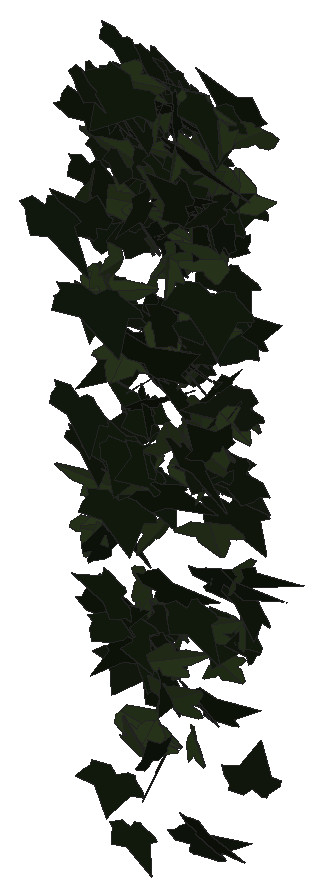
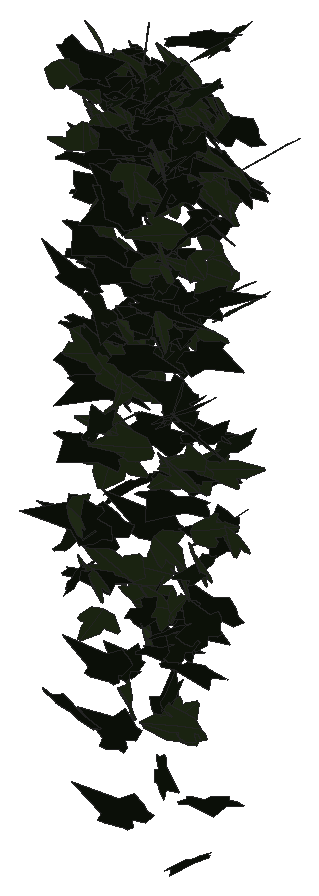
# SketchUp Ruby script. Lengths in millimetres.
U = 1.mm
M = Sketchup.active_model
def pt(a) = Geom::Point3d.new(a.map { |v| v * U })
def face(e, loops, mat)
  f = e.add_face(loops[0].map { |a| pt(a) })
  loops[1..].each { |l| e.add_face(l.map { |a| pt(a) }).erase! }
  f.material = f.back_material = mat if mat
  f
end
# faces: each face lists its corners as indices into pts; further lists are holes
def faces(e, pts, list, mat = nil) = list.each { |f| face(e, (f[0].is_a?(Array) ? f : [f]).map { |l| l.map { |i| pts[i] } }, mat) }
# xy, xz, yz: faces in a plane at the given z, y or x. An outline is a flat list of corners, or four numbers for a rectangle; further outlines are holes
def ring(l) = l.size == 4 ? [[l[0], l[1]], [l[2], l[1]], [l[2], l[3]], [l[0], l[3]]] : l.each_slice(2).to_a
def flat(e, list, mat, &to3) = list.each { |f| face(e, (f[0].is_a?(Array) ? f : [f]).map { |l| ring(l).map { |u, v| to3.(u, v) } }, mat) }
def xy(e, z, list, mat = nil) = flat(e, list, mat) { |x, y| [x, y, z] }
def xz(e, y, list, mat = nil) = flat(e, list, mat) { |x, z| [x, y, z] }
def yz(e, x, list, mat = nil) = flat(e, list, mat) { |y, z| [x, y, z] }
def lines(e, pts, list) = list.each { |a, b| e.add_line(pt(pts[a]), pt(pts[b])) }
# prism: a flat outline (further loops are holes) pulled along v
def prism(e, loops, v, mat = nil)
  f = face(e, loops, mat); d = Geom::Vector3d.new(v.map { |x| x * U })
  f.pushpull(f.normal.samedirection?(d) ? d.length : -d.length)
end
def box(e, o, s, mat = nil) = prism(e, [[o, [o[0] + s[0], o[1], o[2]], [o[0] + s[0], o[1] + s[1], o[2]], [o[0], o[1] + s[1], o[2]]]], [0, 0, s[2]], mat)
def at(x, y, z, deg = 0) = Geom::Transformation.translation(pt([x, y, z])) * Geom::Transformation.rotation(ORIGIN, Z_AXIS, deg.degrees)
def axes(o, x, y, z) = Geom::Transformation.new([*x, 0, *y, 0, *z, 0, *pt(o).to_a, 1])
def part(name) = M.definitions.add(name)
# library, detail: a bought-in or finely detailed component or shape, given as its bounding box
def library(name, o, s) = part(name).tap { |d| box(d.entities, o, s) }
def detail(e, o, s) = box(e.add_group.entities, o, s)
def put(e, d, t, mat = nil) = e.add_instance(d, t).tap { |i| i.material = mat if mat }
def group(e, t, mat = nil) = e.add_group.tap { |g| g.transformation = t; g.material = mat if mat }.entities
root = M.entities
M.materials.add("efeu1").color = [18, 25, 13]
M.materials.add("efeu2").color = [43, 57, 29]
c1 = part("ivyleaf_9")
p = [[39.1,54.8,31.7],[34.5,51.8,30.2],[-5.3,25.2,17.3],[-17.9,28.3,20.9],[-21.6,21.7,17],[-20.2,4.3,5.3],
  [-22.9,-0.3,2.5],[-17.1,-4,-0.6],[-2,-2.1,-1.2],[-0.7,-15.4,-10.1],[16.6,-22.3,-16.7],[21.1,-15.1,-12.5],
  [32.7,-10.7,-11],[46.1,-1.8,-6.6],[30.8,11.2,3.8]]
faces(c1.entities,p,[[0,1,2,3,4,5,6,7,8,9,10,11,12,13,14]],"efeu1")
c2 = part("ivyleaf_10")
p = [[0,12.8,-0.8],[-1.5,51.3,-10.9],[-4.9,51,-11.6],[-13.6,26.5,-7.3],[-13.2,15.9,-4.6],[-21.1,19.3,-7.2],
  [-29.5,16.3,-8.3],[-29.2,8.3,-6.2],[-19.7,-9.8,0.5],[-7.6,-13,4],[1,-12.2,5.8],[-0.4,51.1,-11.1],
  [-1.5,51.1,-10.9],[1,-12.4,5.9],[16.9,-12.4,3.5],[35.1,9.1,-5.1],[35,12.9,-6.1],[20.5,16.4,-4.9],
  [15.8,15,-3.8],[15.3,27.6,-7.1],[12.8,31.3,-7.8]]
faces(c2.entities,p,[[0,1,2,3,4,5,6,7,8,9,10],[11,12,0,13,14,15,16,17,18,19,20]],"efeu2")
put(root,c1,axes([3148,691.4,1357.3],[-1.09848,-0.61121,-0.72388],[0.90904,0.5443,-0.84042],[1.55717,-0.74891,-0.02003]))
put(root,c1,axes([3099.4,712.5,1161.4],[-0.04032,-1.07026,0.20723],[-0.0125,-0.20714,-1.07047],[2.07471,-0.02205,-0.00242]))
put(root,c1,axes([3032,722.5,1449.5],[0.63761,-1.12764,-0.34099],[-0.10545,0.33903,-1.17561],[2.23961,0.337,0.04172]))
put(root,c2,axes([3239.9,749.2,1415.5],[0.02125,0.68623,-0.62586],[-0.04877,-0.62544,-0.68623],[-1.76696,0.02552,0.01141]))
put(root,c1,axes([3194.2,748.7,1503.5],[-1.17443,0.48349,-0.48625],[0.73727,-0.29397,-0.78391],[-1.07685,-0.72857,-0.00639]))
put(root,c1,axes([3272.7,736.2,1533.3],[-0.8878,0.19774,-0.78509],[-1.49185,0.11635,0.49506],[0.38545,0.90577,0.10781]))
put(root,c1,axes([3175.7,773.9,1222.5],[-0.44551,-0.12491,0.99895],[1.62914,-0.56451,0.13],[1.00847,0.85676,0.2313]))
put(root,c1,axes([3253.8,772.5,840.3],[0.29351,-0.90626,-0.43034],[-0.16178,0.42203,-0.91922],[1.90251,0.1757,-0.01177]))
put(root,c1,axes([3088.2,761.2,1424.8],[-0.46198,0.35449,0.80046],[-0.83868,0.66827,-0.42959],[-1.43967,-0.50306,-0.00661]))
put(root,c1,axes([3063.1,778.3,1657.5],[0.90349,-0.93415,-0.35024],[-0.25619,0.32435,-1.04754],[1.88137,0.49278,0.02555]))
put(root,c1,axes([3108.5,793.1,802.7],[0.10206,-0.93985,-0.20129],[0.12799,-0.19744,0.93979],[-1.8248,-0.06641,0.05466]))
put(root,c1,axes([3124.6,800,1646.3],[-1.33312,-0.81117,0.30777],[-0.35091,-0.24734,-1.07154],[1.61349,-0.72401,0.02124]))
put(root,c2,axes([3277,792.5,1420.5],[0.89623,0.07208,-0.78678],[-1.49317,-0.06543,-0.47557],[-0.17745,0.9146,0.02799]))
put(root,c2,axes([3207.7,792.5,668.4],[-1.45962,-0.06032,0.58543],[1.11508,0.01263,0.76884],[-0.10585,0.96475,0.02654]))
put(root,c1,axes([3188.6,813.3,681.3],[0.36799,-0.32379,-0.95206],[1.23033,-0.70261,0.37024],[-1.46603,-0.67093,0.07174]))
put(root,c2,axes([3200.4,811.8,1398.7],[0.20071,-0.42785,0.89084],[0.32043,-0.87502,-0.44019],[1.85335,0.19762,-0.02037]))
put(root,c1,axes([3271.3,806.9,1097.5],[0.4774,0.30872,0.88717],[-1.31395,-0.56208,0.3908],[1.21229,-0.73079,0.0742]))
put(root,c1,axes([3218.8,804.7,1078.1],[0.96684,-0.9688,0.10046],[0.09693,-0.08672,-1.0939],[1.85117,0.51053,0.00481]))
put(root,c2,axes([3156.7,808.8,1496.4],[-0.24848,-0.06951,1.03991],[1.78685,-0.46289,0.08693],[0.86124,0.94032,0.11967]))
put(root,c1,axes([3203.5,791.6,1287.1],[-0.51143,0.05826,-0.9062],[-1.71549,0.09747,0.27355],[0.20954,0.94016,0.0278]))
put(root,c1,axes([3264.3,811.5,1344.9],[-1.0371,-0.88274,-0.40095],[0.4247,0.3334,-1.0373],[1.79567,-0.58869,0.01376]))
put(root,c2,axes([3081.2,820.5,1337.4],[-0.03831,0.03747,0.8963],[0.47235,-0.8613,0.04159],[1.6407,0.24884,0.00896]))
put(root,c1,axes([3173,815.5,1390.4],[0.03374,-0.02831,0.98933],[0.79772,-0.89616,-0.03315],[1.7064,0.4195,-0.00406]))
put(root,c2,axes([3051.7,816.1,1311],[0.85802,-0.35978,0.67627],[1.14747,-0.31739,-0.57078],[0.8993,0.74824,0.08306]))
put(root,c1,axes([3036.7,823.7,1255.8],[-0.31691,-0.83164,0.26203],[-0.10244,-0.25646,-0.84814],[1.65632,-0.17498,-0.00232]))
put(root,c1,axes([3140.3,830.4,1011.4],[-0.57944,-0.40887,0.87701],[-0.74051,-0.79006,-0.50341],[1.68616,-0.48748,0.0803]))
put(root,c2,axes([3188.2,795,722.8],[-0.15978,-0.32421,0.94485],[0.70743,0.86995,0.33153],[-1.76463,0.37812,0.04736]))
put(root,c1,axes([3284.6,810.4,1499.4],[-1.11102,0.68743,-0.20394],[0.25146,-0.15535,-0.90186],[-1.34131,-0.59853,-0.00015]))
put(root,c1,axes([3020.5,835.2,1001.4],[-0.08767,-0.80776,0.5954],[0.1958,-0.59669,-0.80155],[1.89976,0.02422,0.11009]))
put(root,c1,axes([3229.5,826.6,441],[0.54603,-0.41934,0.71364],[0.83487,-0.56347,-0.50746],[1.3359,0.52354,0.02545]))
put(root,c1,axes([3084.2,824.3,936.9],[-0.74249,-0.83718,-0.37572],[0.27869,0.34623,-0.92354],[1.72405,-0.41652,-0.01252]))
put(root,c2,axes([3169.2,811.5,1261.3],[0.56052,0.80983,0.27461],[0.20124,0.25372,-0.86164],[-1.61498,0.31269,-0.01206]))
put(root,c1,axes([3102.9,826.8,1021.5],[-1.48522,-0.20119,-0.38935],[0.72941,0.07237,-0.80557],[0.40456,-0.86911,0.02305]))
put(root,c2,axes([3055.3,826.7,957],[-0.50076,-0.05485,-0.84838],[-1.5783,-0.17897,0.26877],[-0.35623,0.87002,0.0018]))
put(root,c2,axes([3187.8,832.2,1550.4],[-0.00871,0.65938,-0.65939],[-0.13524,-0.65773,-0.65722],[-1.76959,0.04702,0.05347]))
put(root,c2,axes([3032.1,816.5,1449.1],[0.03873,-0.99592,-0.42809],[0.11975,0.42852,-0.99395],[2.05964,-0.00619,0.06584]))
put(root,c1,axes([3200.2,817.5,1443.3],[-0.67275,0.83089,-0.13837],[0.10765,-0.1263,-0.90296],[-1.59952,-0.35797,-0.00257]))
put(root,c2,axes([3274.8,816.8,1073.7],[0.3277,-0.05341,0.90413],[-1.69,0.17123,0.17922],[-0.33935,-0.90431,-0.01946]))
put(root,c1,axes([3197.4,810.1,1632],[0.50681,-0.22295,-0.94817],[-1.4527,0.56287,-0.34672],[1.15159,0.80816,-0.02009]))
put(root,c1,axes([3156.5,826.7,814.8],[0.26163,-0.08827,0.88895],[1.40149,-0.49797,-0.16332],[0.96249,0.7491,-0.00382]))
put(root,c1,axes([3191.8,810.2,1482],[1.32216,0.55374,0.20711],[0.31203,0.12659,-0.88838],[-1.08105,0.71378,-0.00312]))
put(root,c1,axes([3186.8,827.5,1552.9],[1.58032,-0.52072,0.48441],[0.79507,-0.24554,-0.98004],[1.09544,0.92943,0.01248]))
put(root,c1,axes([3099.7,838.4,1182],[1.22544,-0.25384,-0.75639],[1.39495,-0.19579,0.68964],[-0.59987,-0.97385,0.05851]))
put(root,c1,axes([3285.3,812.6,1441.6],[0.26022,-0.08442,0.91084],[-0.26081,0.90868,0.10479],[-1.7213,-0.15045,0.12182]))
put(root,c1,axes([3091.9,839.6,695.2],[-0.25426,0.27227,-0.80449],[0.3543,-0.78519,-0.29666],[-1.57711,-0.22029,0.06306]))
put(root,c2,axes([3110.2,845,1392.7],[-0.51743,-0.16957,1.02457],[1.56141,-0.68442,0.10443],[1.21182,0.80946,0.30292]))
put(root,c1,axes([3155.1,817.3,982.5],[0.0257,0.1341,-0.89414],[0.52498,0.85099,0.1318],[1.63872,-0.27473,-0.0282]))
put(root,c1,axes([3114,822.9,1227.1],[1.53416,0.39429,-0.53653],[-0.93512,-0.21633,-0.89717],[-0.85521,0.94385,0.01851]))
put(root,c1,axes([3123.1,828,1387.6],[-1.26853,0.56479,0.32275],[-0.48523,0.19832,-0.87354],[-1.13899,-0.71351,0.01268]))
put(root,c2,axes([3166.5,841.7,1051.8],[-0.82199,-0.82846,-0.30957],[-0.28298,-0.27159,0.93426],[-1.65924,0.45674,-0.00598]))
put(root,c1,axes([3071.7,847.3,1155.3],[-0.08561,0.08958,-0.88875],[0.18329,-0.88421,-0.094],[-1.69014,-0.10043,0.03482]))
put(root,c2,axes([3084.1,836.3,1176.7],[1.51571,0.3624,-0.22264],[-0.38648,-0.09129,-0.87498],[-0.71127,0.82188,0.00098]))
put(root,c1,axes([3131.6,843.6,520.5],[0.53627,0.37491,0.77182],[-0.8286,-0.63757,0.46864],[1.40723,-0.51828,-0.01819]))
put(root,c1,axes([3018,839.5,1463.6],[-0.89889,-0.013,-0.75126],[1.42369,0.07519,-0.47159],[0.13428,-0.8842,-0.02906]))
put(root,c2,axes([3048,823.7,1276.7],[0.53546,0.15131,-1.02625],[1.82124,0.37262,0.31728],[0.76213,-0.99675,-0.03717]))
put(root,c1,axes([3206.1,833.6,1228.6],[-0.68489,0.53399,0.64734],[0.72924,-0.52209,0.64367],[1.42089,0.52534,-0.01832]))
put(root,c2,axes([3207,840.9,1086.5],[-0.00156,-0.2175,0.94094],[1.82422,-0.11521,-0.0258],[0.2247,0.93386,0.21596]))
put(root,c1,axes([3303,837.1,1056],[-0.1535,-0.02592,-1.05543],[-1.77978,-0.48951,0.08348],[-0.93253,0.93851,0.0144]))
put(root,c2,axes([3020.6,840.6,867.1],[1.41101,-0.46828,0.11897],[0.19326,-0.06201,-0.87689],[0.899,0.74831,0.00178]))
put(root,c2,axes([3279.4,823,1593.2],[0.7223,-0.12595,0.85868],[-1.0972,0.66396,0.35219],[-1.23465,-0.66372,0.18937]))
put(root,c1,axes([3011.3,840.2,1537.7],[-0.58251,0.12731,0.95543],[1.49699,-0.54641,0.32478],[1.06029,0.8414,0.06636]))
put(root,c2,axes([3208.4,842,1264.8],[0.75904,-0.19884,-0.90022],[1.64876,-0.25468,0.44005],[-0.60018,-0.95111,0.07037]))
put(root,c1,axes([3040.4,820.9,845],[0.19601,0.1337,1.01729],[1.32206,0.74337,-0.16803],[-1.43716,0.70206,-0.01582]))
put(root,c2,axes([3049.6,836.3,1424.3],[-0.50917,-0.08974,0.92934],[1.65127,0.33321,0.28194],[-0.6564,0.90786,-0.01162]))
put(root,c1,axes([3070.5,842.8,727],[-0.2822,-0.74749,-0.57441],[0.41705,0.53822,-0.75695],[1.745,-0.24951,0.08802]))
put(root,c2,axes([3159.4,853.4,655.9],[0.36921,-0.80251,0.49862],[0.22163,-0.48483,-0.82562],[1.78443,0.22626,-0.00062]))
put(root,c1,axes([3062.8,848.1,1603.8],[-1.12509,0.16505,-0.63443],[1.17807,-0.14072,-0.61339],[-0.41077,-0.85567,-0.0215]))
put(root,c2,axes([3063.5,844.2,1437],[1.79211,-0.26869,-0.48567],[-0.8916,0.12818,-0.97921],[0.56651,1.05172,-0.00474]))
put(root,c1,axes([3053.3,863.3,1255.6],[-0.1669,-0.5801,-0.82183],[-0.01178,-0.82462,0.58273],[-1.91447,0.05565,0.06806]))
put(root,c1,axes([3054.3,830.3,1379.4],[0.21308,-0.12772,-0.87621],[-0.14631,0.87845,-0.13787],[1.67887,0.09277,0.09919]))
put(root,c1,axes([3073,842.9,1004.7],[-1.1688,-0.59294,0.28239],[0.40465,0.1863,0.85355],[-1.18261,0.64976,0.01297]))
put(root,c1,axes([3274.7,858.6,1264.6],[-0.54401,-0.45618,-0.90021],[-0.78855,-0.80009,0.53701],[-1.75137,0.50194,0.03784]))
put(root,c1,axes([3252.4,849.3,1053.9],[-1.47449,0.23162,-0.36199],[0.6657,-0.0937,-0.80857],[-0.47519,-0.84999,-0.00951]))
put(root,c1,axes([3033.6,848.7,722.3],[-0.25491,0.09954,0.9014],[1.23283,-0.62719,0.16551],[1.20794,0.66112,0.0213]))
put(root,c1,axes([3085,836.8,1401],[-1.13867,0.58624,0.31908],[0.4534,-0.21271,0.83752],[1.18662,0.64383,-0.01383]))
put(root,c1,axes([3129.5,866.2,1251.4],[0.93687,-0.85042,-0.4558],[0.68274,-0.31371,0.97273],[-1.70471,-0.59301,0.13908]))
put(root,c2,axes([3204.7,852.2,1536.4],[-0.30219,-0.08567,1.02244],[-1.82264,-0.35892,-0.17879],[0.70077,-0.97045,-0.02413]))
put(root,c1,axes([3105.6,842.2,1129.4],[0.38507,0.86361,0.15474],[-0.09303,-0.14746,0.88689],[1.66721,-0.20769,0.01375]))
put(root,c1,axes([3084.6,864.8,1563],[-0.18898,-0.82758,0.41164],[0.33627,-0.42337,-0.80854],[1.7267,-0.00812,0.20251]))
put(root,c2,axes([3077.5,859.6,1619],[0.59979,-0.26489,-0.90917],[1.33262,-0.57992,0.41167],[-1.21338,-0.76785,0.00272]))
put(root,c2,axes([3125.5,862.4,1584.3],[0.80852,-0.62316,0.5523],[0.64367,-0.43745,-0.75371],[1.44816,0.54235,0.02665]))
put(root,c1,axes([3132.8,860.9,1229.7],[0.75214,-0.64198,0.51276],[0.67123,-0.38135,-0.74928],[1.41231,0.52314,0.08304]))
put(root,c2,axes([3106.8,846.8,525],[-1.14631,0.5595,-0.36444],[-0.5126,0.24553,0.82208],[1.16285,0.65978,0.00312]))
put(root,c1,axes([3236.9,847.4,1044.9],[0.01688,-0.57967,-0.91706],[0.51885,0.88886,-0.5592],[1.99854,-0.22587,0.15292]))
put(root,c2,axes([3044.1,872.3,873.7],[-0.18463,0.03472,0.93901],[-0.23888,-0.93602,0.02164],[1.77232,-0.12254,0.10074]))
put(root,c2,axes([3258.3,846.5,1295.2],[-0.42523,-0.76212,-0.59809],[0.36332,0.56712,-0.79397],[1.80763,-0.29327,0.01889]))
put(root,c1,axes([3237.7,873.8,1451.7],[-0.42162,-0.82284,0.36012],[-0.17519,-0.34816,-0.85214],[1.70043,-0.23989,0.0015]))
put(root,c1,axes([3182.5,870.2,1513],[-0.19489,-0.94627,0.07143],[-0.0095,-0.0713,-0.95179],[1.80604,-0.10248,0.0027]))
put(root,c2,axes([3169.8,871.5,1469.9],[0.58916,-0.37685,0.75157],[0.9217,-0.57476,-0.48767],[1.30801,0.57475,0.00511]))
put(root,c1,axes([3105.7,855.8,1592.1],[1.40563,-0.2124,0.4587],[0.84346,-0.11856,-0.76846],[0.46274,0.86129,0.00734]))
put(root,c1,axes([3143.7,870.8,1184.6],[0.62085,-0.63434,0.56384],[0.44542,-0.5134,-0.713],[1.55263,0.40094,-0.02092]))
put(root,c2,axes([3106.5,854.4,796.9],[0.82241,-0.80605,-0.48884],[-0.33384,0.45961,-0.91291],[1.76281,0.46309,0.05517]))
put(root,c1,axes([3220.3,873.1,1614],[-0.49748,-1.01728,-0.03229],[0.01648,0.03112,-1.05033],[1.93699,-0.26153,0.00064]))
put(root,c2,axes([3135.6,859.5,1590.4],[1.02429,-0.65135,-0.26115],[-0.27666,0.21849,-0.84454],[1.30662,0.55688,0.0259]))
put(root,c2,axes([3227.1,857.6,928.6],[-1.59016,-0.50603,-0.18202],[0.29431,0.09602,-0.97681],[0.98026,-0.84971,-0.00199]))
put(root,c2,axes([3264.7,849,1126.9],[0.1426,0.79738,0.51971],[0.06277,0.51883,-0.80078],[-1.81036,0.0808,0.01317]))
put(root,c1,axes([3060.7,869,1612],[-0.15584,-0.91483,-0.23042],[0.05705,0.22865,-0.91844],[1.79458,-0.08671,0.00919]))
put(root,c1,axes([3093.9,874.4,953.4],[-1.22073,-0.55624,0.03278],[-0.04578,-0.02229,-0.84901],[1.05948,-0.64186,0.00108]))
put(root,c1,axes([3131.9,878.5,1129.2],[0.33649,-0.87178,0.44567],[0.26842,-0.42548,-0.88823],[1.84397,0.22102,0.04797]))
put(root,c2,axes([3081.2,852.3,957.9],[-0.96001,-0.44969,-0.84006],[1.21341,0.5471,-0.67569],[1.3477,-0.81291,0.00996]))
put(root,c2,axes([3063.4,858.6,1495.2],[0.10711,-0.01039,0.99452],[-1.87733,0.12679,0.05715],[-0.24205,-0.98801,-0.00313]))
put(root,c2,axes([3212.5,881.8,1000.9],[0.30462,-0.49896,0.81623],[0.42544,-0.78516,-0.5238],[1.77031,0.27455,-0.01457]))
put(root,c1,axes([3060.9,872.1,1612.1],[-1.20176,0.09243,-0.60215],[1.12769,-0.10835,-0.63798],[-0.26942,-0.86577,0.01556]))
put(root,c1,axes([3282.1,872.2,1140.6],[-1.4112,-0.04215,0.44705],[-0.85123,-0.00721,-0.74252],[0.07579,-0.8658,-0.01558]))
put(root,c1,axes([3159.2,868,1257.6],[1.20713,-0.34664,0.57854],[0.95845,-0.28486,-0.72278],[0.85381,0.80985,-0.0066]))
put(root,c2,axes([3164.7,870,1450.2],[-1.18883,0.0604,-0.75787],[-1.44662,-0.02901,0.62418],[0.03039,0.98168,0.06508]))
put(root,c1,axes([3108.6,868.4,1198.9],[1.44661,-0.39648,0.29598],[0.49928,-0.13706,-0.85728],[0.79839,0.80409,-0.00018]))
put(root,c1,axes([3246.1,848.6,1166.5],[0.16897,0.71867,0.61151],[0.1303,0.60768,-0.72412],[-1.79118,0.112,0.00501]))
put(root,c2,axes([3248.7,870.5,1508],[1.382,-0.72293,-0.12259],[-0.13676,0.10154,-1.02444],[1.38881,0.72939,0.02111]))
put(root,c1,axes([3225.7,879,1375.3],[0.96986,0.22223,0.84296],[-1.46209,-0.34706,0.55591],[0.78425,-0.92185,-0.00607]))
put(root,c1,axes([3034.9,887.5,1557.9],[0.03908,-0.73537,0.56993],[-0.01775,-0.57021,-0.73539],[1.7706,0.01051,-0.01995]))
put(root,c1,axes([3106.2,866.7,1477.5],[-0.26339,0.22561,0.8065],[-1.33853,0.41247,-0.23607],[-0.86529,-0.70673,0.11968]))
put(root,c2,axes([3174.2,873.7,1606],[-0.0944,0.00486,-0.90035],[1.63504,-0.2696,-0.04878],[-0.51282,-0.86047,0.0102]))
put(root,c1,axes([3057.4,875.4,1568.8],[-1.36606,0.27318,-0.35069],[0.64422,-0.09588,-0.76749],[-0.54843,-0.79309,-0.02801]))
put(root,c1,axes([3083,888.1,1079.4],[0.34647,-0.15233,-0.90399],[1.34867,-0.56132,0.23729],[-1.10688,-0.73162,0.00616]))
put(root,c2,axes([3197.2,869.8,749.6],[-1.19274,-0.30094,0.6971],[1.21052,0.28557,0.6951],[-0.78921,0.89283,0.01264]))
put(root,c1,axes([3083.7,878.4,1561.7],[-0.25442,-0.94281,-0.35649],[0.18901,0.34554,-0.9511],[1.90901,-0.15987,0.04666]))
put(root,c2,axes([3103.6,878.1,1289.8],[0.5209,-0.76664,-0.23931],[0.1543,-0.22515,0.81403],[-1.52069,-0.28545,0.00062]))
put(root,c1,axes([3257.3,876.9,1139.9],[-0.99973,0.5187,-0.44741],[0.56591,-0.33527,-0.73779],[-1.17446,-0.60308,0.02535]))
put(root,c2,axes([3074.4,856.2,960.2],[-0.0229,-0.38747,0.96378],[0.05174,0.9634,0.38766],[-1.97628,0.02971,-0.00102]))
put(root,c1,axes([3069.8,866.9,1537.2],[1.42122,-0.11122,-0.47303],[-0.88584,0.08547,-0.75487],[0.26571,0.87983,0.01353]))
put(root,c2,axes([3167.4,887.7,547.1],[0.22037,-0.11647,0.92285],[1.32418,-0.60639,-0.16383],[1.17497,0.70524,0.01155]))
put(root,c2,axes([3170.4,868.5,1147.1],[0.40976,-0.80851,0.35731],[-0.00132,0.3676,0.83222],[-1.68232,-0.19722,0.08638]))
put(root,c2,axes([3227.1,880.7,1500.8],[-0.39561,-0.89241,0.2302],[0.00526,-0.23659,-0.91467],[1.75402,-0.20057,0.05466]))
put(root,c2,axes([3033.3,859.9,1580.3],[-0.38709,-0.20216,-0.98043],[1.30495,0.7008,-0.28674],[1.38813,-0.71518,-0.00384]))
put(root,c1,axes([3100.5,880,690.6],[-0.87332,-0.06523,-0.85105],[1.58611,0.17448,-0.46272],[0.3509,-0.951,-0.02653]))
put(root,c1,axes([3134.3,858.7,1589.5],[0.95335,0.40394,0.56191],[0.71034,0.42644,-0.63928],[-1.10911,0.62033,0.07357]))
put(root,c1,axes([3141.1,871.4,1508.1],[0.41935,-0.57747,-0.68822],[0.46665,0.72037,-0.52594],[1.64492,-0.05715,0.32466]))
put(root,c2,axes([3119,885.6,1495.8],[0.16882,-0.87143,0.33371],[0.08431,-0.3309,-0.87588],[1.77395,0.09866,0.00987]))
put(root,c1,axes([3066.4,885.9,645.9],[-1.37329,-0.40686,-0.14062],[0.2364,0.066,-0.82836],[0.78443,-0.73217,0.00347]))
put(root,c2,axes([3138.9,889.6,691.5],[0.54017,-0.62548,0.57367],[0.50051,-0.51032,-0.68651],[1.53579,0.38631,0.02196]))
put(root,c1,axes([3062.6,868.5,1491.2],[0.48476,-0.54872,-0.85661],[-0.30208,0.8508,-0.59219],[1.91238,0.27348,0.12359]))
put(root,c1,axes([3195.7,874.4,1441.3],[-0.3702,-0.02702,0.88712],[1.66102,-0.17085,0.18616],[0.30693,0.89198,0.06253]))
put(root,c1,axes([3147.7,889.9,1466.4],[-1.72751,-0.27954,0.29998],[-0.54718,-0.08564,-0.94975],[0.55641,-0.95213,-0.00265]))
put(root,c1,axes([3080.1,866,1075.6],[0.44392,0.84885,-0.28298],[0.13865,0.27345,0.88031],[1.69729,-0.24435,0.0021]))
put(root,c1,axes([3026,888.5,435.1],[-0.90851,-0.66946,-0.11372],[0.13134,0.09046,-0.82221],[1.28567,-0.48231,0.00364]))
put(root,c1,axes([3089.6,880.1,1049.2],[-1.49317,0.3526,0.08163],[-0.14448,0.03021,-0.86014],[-0.67349,-0.78821,0.00355]))
put(root,c1,axes([3142.7,886,1227.3],[-1.38722,0.02884,0.51759],[-0.98611,-0.01249,-0.72896],[-0.03097,-0.89388,0.02688]))
put(root,c1,axes([3099.2,885.2,1049],[-0.75033,-0.86849,0.10666],[0.08337,0.09724,0.95379],[-1.66324,0.39667,-0.00031]))
put(root,c2,axes([3197.5,871,1550.3],[0.58517,-0.52133,-0.65044],[-0.46316,0.60694,-0.6015],[1.51736,0.38631,0.06725]))
put(root,c2,axes([3086,878.4,516],[1.53144,0.10699,-0.20891],[0.39234,0.03455,0.81172],[0.21357,-0.83063,0.00685]))
put(root,c2,axes([3180.6,871.9,1086.7],[-0.36234,-0.733,-0.64026],[0.41278,0.60404,-0.75602],[1.80572,-0.28517,0.04434]))
put(root,c1,axes([3163.5,896.2,610.7],[0.27611,-0.47662,0.66592],[0.44391,-0.62423,-0.49759],[1.49399,0.27356,0.02478]))
put(root,c1,axes([3045.8,881.9,1386.2],[0.53809,-0.72917,-0.45243],[-0.33134,0.4177,-0.78201],[1.59922,0.33189,-0.00979]))
put(root,c1,axes([3013.1,879.8,1484.9],[0.75256,-0.67732,-0.47211],[-0.06145,0.51038,-0.75926],[1.57012,0.34461,0.19657]))
put(root,c2,axes([3163.4,895,1393.2],[-0.35089,0.10656,0.9668],[1.53869,-0.5303,0.21262],[1.02919,0.82915,0.01174]))
put(root,c2,axes([3190,884.7,993.3],[0.07829,-0.10916,0.8964],[1.71248,0.08079,-0.03146],[-0.14524,0.8937,0.11234]))
put(root,c2,axes([3184.8,886.9,1085.7],[-0.81757,-0.05843,0.8945],[1.70315,0.02971,0.43171],[-0.09917,0.99186,0.03976]))
put(root,c1,axes([3098.4,895.6,667.7],[-0.92556,-0.72464,-0.09334],[0.09629,0.07845,-0.8727],[1.38719,-0.48894,-0.0017]))
put(root,c1,axes([3129.8,901.5,729.1],[-0.10043,-0.10494,-0.85907],[0.1353,-0.85828,0.10048],[-1.64156,-0.06432,0.06084]))
put(root,c1,axes([3206.4,898.5,1586.4],[-0.88765,-0.9382,-0.16477],[0.11138,0.15489,-1.04761],[1.80949,-0.46977,-0.01634]))
put(root,c1,axes([3205.8,886.6,818.2],[0.69925,-0.1867,0.87126],[1.57396,-0.27934,-0.40861],[0.63123,0.90335,0.05372]))
put(root,c1,axes([3183,888.5,1276.9],[-0.65317,-0.4281,-0.67532],[0.86198,0.50155,-0.54811],[1.25408,-0.5677,0.02501]))
put(root,c1,axes([3082,904.2,590.7],[-0.15151,-0.30213,0.75968],[-0.18262,-0.75454,-0.31014],[1.54521,-0.1188,0.03783]))
put(root,c1,axes([3254.4,906,800.5],[-0.09896,-0.82143,0.53342],[0.12516,-0.5359,-0.81883],[1.85985,-0.00764,0.08349]))
put(root,c2,axes([3076.7,903.9,745.9],[-0.002,0.01749,-0.83667],[-0.23969,-0.82714,-0.01713],[-1.57455,0.12589,0.00367]))
put(root,c1,axes([3239,888.9,957.4],[-0.67282,-0.31316,-0.77527],[1.14586,0.48874,-0.47196],[1.10424,-0.69797,0.01737]))
put(root,c2,axes([3060.4,884,544.5],[0.64957,0.13266,0.88613],[1.56814,0.3261,-0.36617],[-0.67002,0.89184,0.00208]))
put(root,c1,axes([3116.6,905.5,1522],[-0.60356,-0.08599,1.04204],[0.44994,-1.06661,-0.01607],[1.93841,0.2208,0.32819]))
put(root,c1,axes([3234.7,900.2,749.7],[-1.31254,-0.57396,-0.11611],[0.18119,0.06711,-0.89719],[1.09965,-0.69613,0.00925]))
put(root,c2,axes([3101.8,896.3,736.2],[-0.71545,0.35119,-0.72693],[1.02042,-0.49089,-0.51442],[-1.14871,-0.6548,-0.00422]))
put(root,c2,axes([3071.6,891.1,1601.5],[1.21892,-0.17967,-0.51993],[-0.97141,0.10351,-0.6645],[0.39046,0.81841,-0.0301]))
put(root,c2,axes([3110.6,889.4,1213],[0.06615,-0.82313,-0.19316],[-0.03143,0.19263,-0.82382],[1.60882,0.03761,-0.00815]))
put(root,c1,axes([3086,906.6,705.4],[-0.60232,-0.66548,0.32812],[-0.21846,-0.30851,-0.73643],[1.39512,-0.33562,0.02634]))
put(root,c2,axes([3238.1,897.1,751.8],[1.35077,-0.65256,-0.03151],[-0.04154,0.02281,-0.96413],[1.2427,0.71007,0.00202]))
put(root,c1,axes([3140.5,908.9,1575.7],[0.02936,-0.12146,0.89187],[0.17827,-0.88694,-0.12241],[1.70378,0.0949,-0.00256]))
put(root,c1,axes([3009.3,906.9,728.7],[1.27368,-0.24845,-0.60284],[1.06642,-0.22261,0.71378],[-0.63459,-0.87277,-0.01045]))
put(root,c2,axes([3235.5,877,1363.2],[-0.0432,0.24114,-0.87397],[-0.00251,0.87423,0.24125],[1.72548,0.00731,-0.02153]))
put(root,c2,axes([3277,900.3,1582.6],[-1.153,-0.47256,0.57757],[-0.87109,-0.35229,-0.76832],[1.12177,-0.75928,-0.00298]))
put(root,c2,axes([3051.4,897.7,961.5],[0.95867,-0.34877,-0.56935],[1.01125,-0.2225,0.60638],[-0.76951,-0.7269,0.08757]))
put(root,c1,axes([3089.3,905.7,1607.2],[-0.96049,0.10336,-0.86624],[1.54001,-0.31856,-0.50943],[-0.62053,-0.95057,0.07653]))
put(root,c2,axes([3033,906.4,1346.3],[-0.16632,-0.70219,0.49403],[0.32165,-0.50094,-0.68211],[1.60205,0.02768,0.18824]))
put(root,c2,axes([3253.4,910.2,850.9],[0.28723,-0.77413,0.62807],[0.20301,-0.61904,-0.78863],[1.88636,0.18449,-0.01076]))
put(root,c1,axes([3108.6,910.6,1616.7],[-0.15698,-0.86156,0.18638],[0.00478,-0.18743,-0.86527],[1.67765,-0.08008,0.0199]))
put(root,c1,axes([3258,915.7,727.4],[-0.21829,-0.20503,0.845],[-0.73175,-0.75251,-0.23477],[1.48429,-0.40114,0.00853]))
put(root,c1,axes([3120.8,902.2,1433.7],[0.84075,-0.55624,0.5064],[-0.59416,0.39873,0.71031],[-1.30252,-0.54093,0.00285]))
put(root,c1,axes([3064.5,885.2,1457.7],[0.11072,-0.19803,-0.85883],[-0.54489,0.80977,-0.20612],[1.58645,0.29195,-0.01086]))
put(root,c1,axes([3142.7,899.6,1386.9],[1.68975,0.35219,-0.14803],[0.24212,0.08058,0.95475],[0.68559,-0.89649,0.02766]))
put(root,c1,axes([3235,909.9,1459.4],[-0.94066,-0.77119,-0.08333],[0.10161,0.06475,-0.91592],[1.47276,-0.49703,0.00997]))
put(root,c2,axes([3126.4,914,1305.7],[-0.30176,-0.1143,0.80153],[-0.14011,-0.81134,-0.13026],[1.53453,-0.09655,0.14573]))
put(root,c1,axes([3185.4,899.6,598],[0.03127,-0.08115,0.8107],[1.40992,-0.33604,-0.04865],[0.64546,0.73796,0.067]))
put(root,c2,axes([3249.5,894.5,1460.4],[1.52412,0.51694,-0.08392],[0.11545,0.06074,0.953],[0.99001,-0.80291,0.01806]))
put(root,c2,axes([3150.4,890.5,987.9],[0.39717,0.06065,0.89339],[1.26387,0.60489,-0.19619],[-1.14324,0.68979,0.09348]))
put(root,c2,axes([3149.6,899.3,1454.4],[-1.17972,-0.61374,-0.08379],[0.11048,0.06046,-0.87229],[1.17371,-0.62257,-0.00211]))
put(root,c1,axes([3078.7,908.8,1636.2],[0.93283,-0.98605,0.00574],[0.0196,-0.00129,-1.10111],[1.87658,0.49017,0.00865]))
put(root,c1,axes([3043.2,916.5,692.5],[0.26213,-0.58989,0.63667],[0.30513,-0.61626,-0.60565],[1.62344,0.21107,0.01103]))
put(root,c2,axes([3082.8,891.4,1370.1],[0.53958,0.20634,0.86985],[1.178,0.61314,-0.34718],[-1.22768,0.67902,0.04917]))
put(root,c1,axes([3150.3,914.9,1153],[-0.20603,-0.07072,-0.82973],[-0.29962,-0.81989,0.09042],[-1.55629,0.16721,0.09244]))
put(root,c2,axes([3229.4,908.8,1124.4],[0.92645,-0.18862,0.73526],[1.35998,-0.18078,-0.51947],[0.48734,0.86307,0.05188]))
put(root,c2,axes([3086.4,915.1,857.5],[-0.11818,-0.8137,0.51781],[-0.0386,-0.51767,-0.81591],[1.83522,-0.06329,0.01619]))
put(root,c1,axes([3092.7,913,473.2],[-0.62505,0.29888,-0.74763],[0.99763,-0.53351,-0.44355],[-1.16314,-0.61821,0.02133]))
put(root,c1,axes([3158.8,901.6,364.2],[0.0694,-0.05868,0.82497],[1.51753,-0.21681,-0.05066],[0.41803,0.79681,0.04697]))
put(root,c1,axes([3213,906.5,1326.4],[-0.91803,-0.19036,-0.79523],[1.36887,0.34043,-0.51776],[0.7403,-0.86554,-0.02875]))
put(root,c1,axes([3159.9,907.3,1508.4],[-0.76413,-0.35129,-0.73442],[1.20683,0.37863,-0.52776],[0.97173,-0.74647,0.07792]))
put(root,c1,axes([3084.3,922,1598.7],[-0.43824,-0.66515,0.52656],[-0.02113,-0.5432,-0.69103],[1.61443,-0.18767,0.13389]))
put(root,c1,axes([3171.1,915.1,1574],[0.13679,-0.90825,-0.00172],[0.01724,-0.00101,0.91105],[-1.7285,-0.07189,0.00895]))
put(root,c1,axes([3252.4,899,1600],[0.17763,-0.12126,0.90251],[-1.12764,0.68085,0.15275],[-1.31606,-0.59973,-0.00907]))
put(root,c2,axes([3104.5,908.6,1429.3],[0.77232,-0.04833,0.8407],[1.59421,-0.0726,-0.4085],[0.16446,0.93069,0.0118]))
put(root,c1,axes([3012.1,920.1,1636.5],[0.07406,-0.8499,0.36099],[0.12061,-0.35801,-0.84969],[1.75325,0.06053,0.04321]))
put(root,c2,axes([3217.5,898.3,682],[-0.70106,-0.58269,-0.4797],[0.58484,0.37175,-0.68754],[1.31198,-0.47708,0.05015]))
put(root,c1,axes([3174,917.9,1028.2],[0.0357,-0.95995,0.10687],[0.02306,-0.10665,-0.96008],[1.83813,0.01998,0.00997]))
put(root,c1,axes([3067,906.4,937.1],[-0.61735,-0.60678,-0.67825],[0.62496,0.5935,-0.688],[1.61533,-0.46152,0.00697]))
put(root,c1,axes([3100.2,920.6,1586.5],[-0.28598,0.0726,0.87994],[-0.95764,-0.7405,-0.02483],[1.38081,-0.49853,0.16503]))
put(root,c1,axes([3234.5,891,836.3],[0.4061,0.50362,-0.77703],[0.55516,0.72023,0.54692],[1.67257,-0.36134,0.00713]))
put(root,c1,axes([3198.3,923.6,1010.2],[-0.01522,-0.53688,0.69339],[0.13754,-0.69147,-0.53456],[1.66333,0.05227,0.05055]))
put(root,c1,axes([3273.3,896.3,501.8],[-1.40581,0.49497,0.09156],[0.13517,-0.05847,0.88911],[0.94842,0.74201,0.00899]))
put(root,c1,axes([3036.1,912,339.8],[0.08728,-0.77951,-0.22466],[-0.02597,0.22425,-0.78086],[1.54373,0.04784,-0.00044]))
put(root,c1,axes([3162.8,905.3,1566],[-1.55191,-0.22777,-0.38594],[-0.71102,-0.09706,0.84661],[-0.47105,0.89691,-0.00639]))
put(root,c1,axes([3009.2,912.3,839.8],[0.83593,-0.67093,-0.0204],[-0.02133,0.01705,-0.80191],[1.27733,0.43937,-0.00004]))
put(root,c2,axes([3101.5,909.2,1513.9],[0.62478,-0.83126,-0.13869],[-0.0392,0.14088,-0.89316],[1.60345,0.32734,0.0322]))
put(root,c1,axes([3237.8,914,1238.2],[-0.19777,0.16615,0.82796],[0.95236,-0.65986,0.19522],[1.29463,0.51079,-0.01713]))
put(root,c2,axes([3021.3,915.7,856.5],[1.12641,-0.73086,0.1577],[0.19185,-0.12129,-0.94045],[1.41,0.60037,0.00198]))
put(root,c1,axes([3182.5,890.2,1377.2],[0.65486,0.49996,0.73401],[0.83009,0.59058,-0.60673],[-1.47238,0.55532,-0.01559]))
